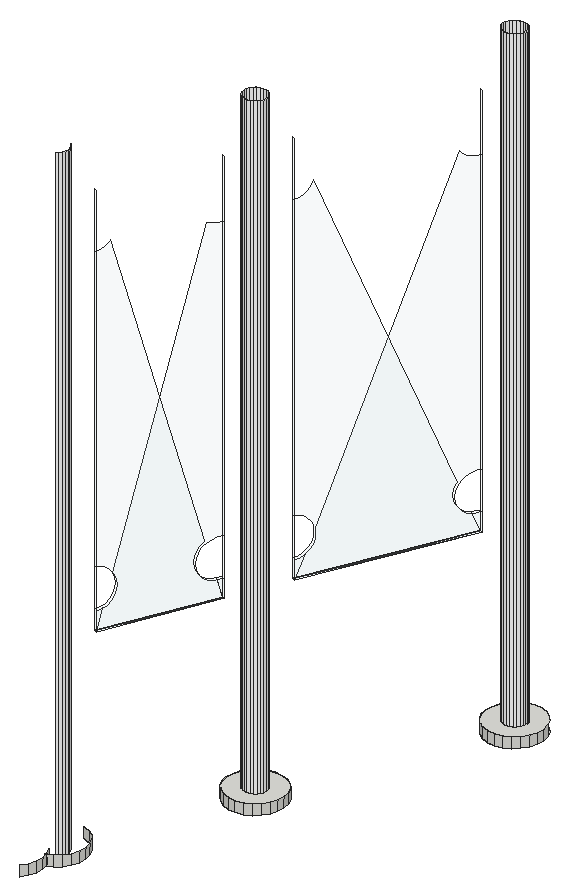
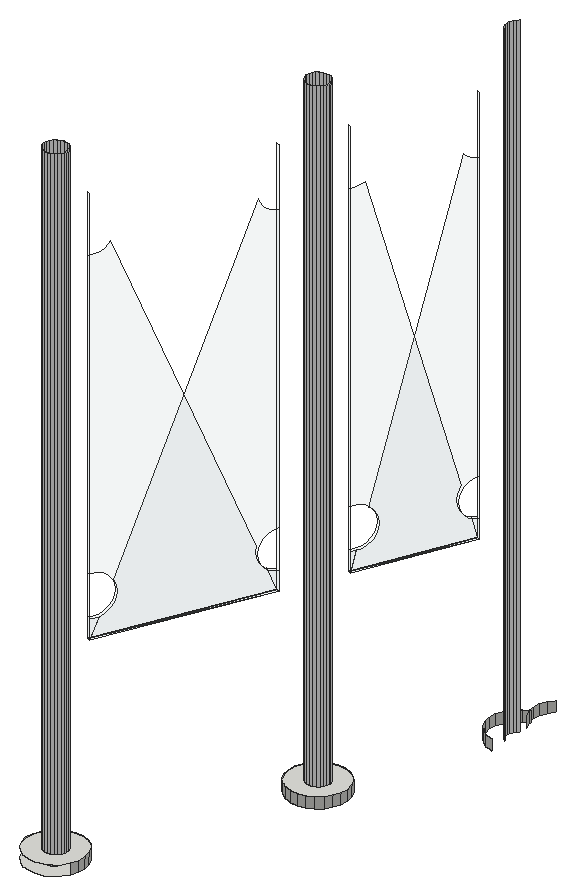
# SketchUp Ruby script. Lengths in inches.
U = 1.inch
M = Sketchup.active_model
def pt(a) = Geom::Point3d.new(a.map { |v| v * U })
def face(e, loops, mat)
  f = e.add_face(loops[0].map { |a| pt(a) })
  loops[1..].each { |l| e.add_face(l.map { |a| pt(a) }).erase! }
  f.material = f.back_material = mat if mat
  f
end
# faces: each face lists its corners as indices into pts; further lists are holes
def faces(e, pts, list, mat = nil) = list.each { |f| face(e, (f[0].is_a?(Array) ? f : [f]).map { |l| l.map { |i| pts[i] } }, mat) }
# xy, xz, yz: faces in a plane at the given z, y or x. An outline is a flat list of corners, or four numbers for a rectangle; further outlines are holes
def ring(l) = l.size == 4 ? [[l[0], l[1]], [l[2], l[1]], [l[2], l[3]], [l[0], l[3]]] : l.each_slice(2).to_a
def flat(e, list, mat, &to3) = list.each { |f| face(e, (f[0].is_a?(Array) ? f : [f]).map { |l| ring(l).map { |u, v| to3.(u, v) } }, mat) }
def xy(e, z, list, mat = nil) = flat(e, list, mat) { |x, y| [x, y, z] }
def xz(e, y, list, mat = nil) = flat(e, list, mat) { |x, z| [x, y, z] }
def yz(e, x, list, mat = nil) = flat(e, list, mat) { |y, z| [x, y, z] }
def lines(e, pts, list) = list.each { |a, b| e.add_line(pt(pts[a]), pt(pts[b])) }
# prism: a flat outline (further loops are holes) pulled along v
def prism(e, loops, v, mat = nil)
  f = face(e, loops, mat); d = Geom::Vector3d.new(v.map { |x| x * U })
  f.pushpull(f.normal.samedirection?(d) ? d.length : -d.length)
end
def box(e, o, s, mat = nil) = prism(e, [[o, [o[0] + s[0], o[1], o[2]], [o[0] + s[0], o[1] + s[1], o[2]], [o[0], o[1] + s[1], o[2]]]], [0, 0, s[2]], mat)
def at(x, y, z, deg = 0) = Geom::Transformation.translation(pt([x, y, z])) * Geom::Transformation.rotation(ORIGIN, Z_AXIS, deg.degrees)
def axes(o, x, y, z) = Geom::Transformation.new([*x, 0, *y, 0, *z, 0, *pt(o).to_a, 1])
def part(name) = M.definitions.add(name)
# library, detail: a bought-in or finely detailed component or shape, given as its bounding box
def library(name, o, s) = part(name).tap { |d| box(d.entities, o, s) }
def detail(e, o, s) = box(e.add_group.entities, o, s)
def put(e, d, t, mat = nil) = e.add_instance(d, t).tap { |i| i.material = mat if mat }
def group(e, t, mat = nil) = e.add_group.tap { |g| g.transformation = t; g.material = mat if mat }.entities
root = M.entities
M.materials.add("Glass_Safety_01").color = [204, 235, 244]
M.materials["Glass_Safety_01"].alpha = 0.1
M.materials.add("[Color_000]").color = [255, 255, 255]
xy(root,321.27,[[[848.125,545.34,848.53,545.42,848.9,545.6,849.2,545.875,849.43,546.22,849.56,546.61,849.58,547.02,849.5,547.42,849.32,547.79,849.05,548.1,848.7,548.32,848.64,548.34,848.3125,548.45,847.9,548.48,847.5,548.4,847.13,548.21,846.82,547.9375,846.6,547.6,846.47,547.21,846.44,546.79,846.53,546.39,846.71,546.02,846.98,545.72,847.33,545.49,847.72,545.36],[848.06,546.28,847.89,546.29,847.76,546.33,847.74,546.34,847.6,546.43,847.49,546.55,847.42,546.7,847.39,546.86,847.4,547.03,847.45,547.18,847.54,547.32,847.66,547.43,847.81,547.5,847.97,547.54,848.13,547.53,848.26,547.48,848.29,547.47,848.43,547.38,848.54,547.26,848.61,547.11,848.64,546.95,848.63,546.79,848.58,546.63,848.49,546.49,848.37,546.39,848.22,546.3125]],[847.39,545.47,847.76,546.33,847.74,546.34,847.6,546.43,847.49,546.55,847.42,546.7,847.39,546.86,847.4,547.03,847.45,547.18,847.54,547.32,847.66,547.43,847.81,547.5,847.97,547.54,848.13,547.53,848.26,547.48,848.64,548.34,848.3125,548.45,847.9,548.48,847.5,548.4,847.13,548.21,846.82,547.9375,846.6,547.6,846.47,547.21,846.44,546.79,846.53,546.39,846.71,546.02,846.98,545.72,847.33,545.49],[847.76,546.33,848.26,547.48,848.13,547.53,847.97,547.54,847.81,547.5,847.66,547.43,847.54,547.32,847.45,547.18,847.4,547.03,847.39,546.86,847.42,546.7,847.49,546.55,847.6,546.43,847.74,546.34],[[853.35,557.32,853.75,557.4,854.12,557.59,854.42,557.86,854.65,558.2,854.78,558.59,854.8,559,854.72,559.41,854.54,559.77,854.26,560.08,853.92,560.31,853.86,560.33,853.53,560.4375,853.12,560.46,852.72,560.38,852.35,560.19,852.04,559.92,851.82,559.58,851.6875,559.1875,851.66,558.78,851.75,558.375,851.93,558.01,852.2,557.7,852.55,557.47,852.94,557.34],[853.28,558.26,853.11,558.27,852.98,558.32,852.96,558.32,852.82,558.41,852.71,558.54,852.64,558.68,852.6,558.85,852.61,559.01,852.67,559.17,852.76,559.3,852.88,559.41,853.03,559.49,853.1875,559.52,853.35,559.51,853.48,559.47,853.51,559.46,853.65,559.37,853.75,559.24,853.83,559.1,853.86,558.9375,853.85,558.77,853.8,558.62,853.71,558.48,853.59,558.37,853.4375,558.3]],[852.61,557.45,852.98,558.32,852.96,558.32,852.82,558.41,852.71,558.54,852.64,558.68,852.6,558.85,852.61,559.01,852.67,559.17,852.76,559.3,852.88,559.41,853.03,559.49,853.1875,559.52,853.35,559.51,853.48,559.47,853.86,560.33,853.53,560.4375,853.12,560.46,852.72,560.38,852.35,560.19,852.04,559.92,851.82,559.58,851.6875,559.1875,851.66,558.78,851.75,558.375,851.93,558.01,852.2,557.7,852.55,557.47],
  [852.96,558.32,852.98,558.32,853.48,559.47,853.35,559.51,853.1875,559.52,853.03,559.49,852.88,559.41,852.76,559.3,852.67,559.17,852.61,559.01,852.6,558.85,852.64,558.68,852.71,558.54,852.82,558.41]])
xy(root,321.27,[[848.06,546.28,848.22,546.3125,848.37,546.39,848.49,546.49,848.58,546.63,848.63,546.79,848.64,546.95,848.61,547.11,848.54,547.26,848.43,547.38,848.29,547.47,848.26,547.48,847.76,546.33,847.89,546.29],[853.28,558.26,853.4375,558.3,853.59,558.37,853.71,558.48,853.8,558.62,853.85,558.77,853.86,558.9375,853.83,559.1,853.75,559.24,853.65,559.37,853.51,559.46,853.48,559.47,852.98,558.32,853.11,558.27]],"[Color_000]")
xy(root,321.86,[[848.125,545.34,848.53,545.42,848.9,545.6,849.2,545.875,849.43,546.22,849.56,546.61,849.58,547.02,849.5,547.42,849.32,547.79,849.05,548.1,848.7,548.32,848.3125,548.45,847.9,548.48,847.5,548.4,847.13,548.21,846.82,547.9375,846.6,547.6,846.47,547.21,846.44,546.79,846.53,546.39,846.71,546.02,846.98,545.72,847.33,545.49,847.72,545.36],[853.35,557.32,853.75,557.4,854.12,557.59,854.42,557.86,854.65,558.2,854.78,558.59,854.8,559,854.72,559.41,854.54,559.77,854.26,560.08,853.92,560.31,853.53,560.4375,853.12,560.46,852.72,560.38,852.35,560.19,852.04,559.92,851.82,559.58,851.6875,559.1875,851.66,558.78,851.75,558.375,851.93,558.01,852.2,557.7,852.55,557.47,852.94,557.34]])
xy(root,331.9,[[844.9,539.5,844.72,539.58,847.47,545.42],[844.72,539.58,847.29,545.5,847.47,545.42],[848.89,548.67,848.71,548.75,852.66,557.32],[848.71,548.75,852.48,557.4,852.66,557.32]],"Glass_Safety_01")
p = [[844.27,534.8,321.27],[844.5,535.14,321.27],[844.5,535.14,321.86],[844.27,534.8,321.86],[844.63,535.53,321.27],[844.63,535.53,321.86],
  [844.66,535.94,321.27],[844.66,535.94,321.86],[844.59,536.27,321.27],[844.57,536.34,321.27],[844.57,536.34,321.86],[844.59,536.27,321.86],
  [844.53,536.25,321.27],[844.9,536.43,321.27],[844.9,536.43,321.86],[844.53,536.25,321.86],[844.39,536.71,321.27],[844.39,536.71,321.86],
  [845.21,536.7,321.27],[845.21,536.7,321.86],[845.4375,537.05,321.27],[845.4375,537.05,321.86],[845.57,537.4375,321.27],[845.57,537.4375,321.86],
  [844.37,537.21,321.27],[844.5,537.32,321.27],[844.5,537.32,357.27],[844.37,537.21,357.27],[844.59,537.46,321.27],[844.59,537.46,357.27],
  [845.59,537.85,321.27],[845.59,537.85,321.86],[844.64,537.62,321.27],[844.64,537.62,357.27],[844.65,537.78,321.27],[844.65,537.78,357.27],
  [844.61,537.94,321.27],[844.61,537.94,357.27],[845.51,538.25,321.27],[845.51,538.25,321.86],[844.54,538.09,321.27],[844.54,538.09,357.27],
  [844.43,538.21,321.27],[844.43,538.21,357.27],[845.32,538.62,321.27],[845.32,538.62,321.86],[845.05,538.93,321.27],[845.05,538.93,321.86],
  [844.71,539.15,321.27],[844.71,539.15,321.86],[844.65,539.17,321.27],[844.32,539.28,321.27],[844.32,539.28,321.86],[847.72,545.36,321.27],
  [848.125,545.34,321.27],[848.125,545.34,321.86],[847.72,545.36,321.86],[848.53,545.42,321.27],[848.53,545.42,321.86],[847.33,545.49,321.27],
  [847.39,545.47,321.27],[847.33,545.49,321.86],[848.9,545.6,321.27],[848.9,545.6,321.86],[846.98,545.72,321.27],[846.98,545.72,321.86],
  [849.2,545.875,321.27],[849.2,545.875,321.86],[846.71,546.02,321.27],[846.71,546.02,321.86],[849.43,546.22,321.27],[849.43,546.22,321.86],
  [846.53,546.39,321.27],[846.53,546.39,321.86],[849.56,546.61,321.27],[849.56,546.61,321.86],[847.6,546.43,321.27],[847.74,546.34,321.27],
  [847.74,546.34,357.27],[847.6,546.43,357.27],[847.76,546.33,321.27],[847.89,546.29,321.27],[847.89,546.29,357.27],[848.06,546.28,321.27],
  [848.06,546.28,357.27],[848.22,546.3125,321.27],[848.22,546.3125,357.27],[848.37,546.39,321.27],[848.37,546.39,357.27],[846.44,546.79,321.27],
  [846.44,546.79,321.86],[847.49,546.55,321.27],[847.49,546.55,357.27],[848.49,546.49,321.27],[848.49,546.49,357.27],[848.58,546.63,321.27],
  [848.58,546.63,357.27],[847.42,546.7,321.27],[847.42,546.7,357.27],[848.63,546.79,321.27],[848.63,546.79,357.27],[849.58,547.02,321.27],
  [849.58,547.02,321.86],[847.39,546.86,321.27],[847.39,546.86,357.27],[846.47,547.21,321.27],[846.47,547.21,321.86],[848.64,546.95,321.27],
  [848.64,546.95,357.27],[847.4,547.03,321.27],[847.4,547.03,357.27],[847.45,547.18,321.27],[847.45,547.18,357.27],[848.61,547.11,321.27],
  [848.61,547.11,357.27],[849.5,547.42,321.27],[849.5,547.42,321.86],[848.54,547.26,321.27],[848.54,547.26,357.27],[846.6,547.6,321.27],
  [846.6,547.6,321.86],[847.54,547.32,321.27],[847.54,547.32,357.27],[847.66,547.43,321.27],[847.66,547.43,357.27],[848.43,547.38,321.27],
  [848.43,547.38,357.27],[847.81,547.5,321.27],[847.81,547.5,357.27],[848.29,547.47,321.27],[848.29,547.47,357.27],[849.32,547.79,321.27],
  [849.32,547.79,321.86],[847.97,547.54,321.27],[847.97,547.54,357.27],[848.13,547.53,321.27],[848.13,547.53,357.27],[848.26,547.48,321.27],
  [846.82,547.9375,321.27],[846.82,547.9375,321.86],[849.05,548.1,321.27],[849.05,548.1,321.86],[847.13,548.21,321.27],[847.13,548.21,321.86],
  [848.7,548.32,321.27],[848.7,548.32,321.86],[847.5,548.4,321.27],[847.5,548.4,321.86],[848.64,548.34,321.27],[848.3125,548.45,321.27],
  [848.3125,548.45,321.86],[847.9,548.48,321.27],[847.9,548.48,321.86],[852.55,557.47,321.27],[852.61,557.45,321.27],[852.94,557.34,321.27],
  [852.94,557.34,321.86],[852.55,557.47,321.86],[853.35,557.32,321.27],[853.35,557.32,321.86],[853.75,557.4,321.27],[853.75,557.4,321.86],
  [854.12,557.59,321.27],[854.12,557.59,321.86],[852.2,557.7,321.27],[852.2,557.7,321.86],[854.42,557.86,321.27],[854.42,557.86,321.86],
  [851.93,558.01,321.27],[851.93,558.01,321.86],[854.65,558.2,321.27],[854.65,558.2,321.86],[851.75,558.375,321.27],[851.75,558.375,321.86],
  [854.78,558.59,321.27],[854.78,558.59,321.86],[852.82,558.41,321.27],[852.96,558.32,321.27],[852.96,558.32,357.27],[852.82,558.41,357.27],
  [852.98,558.32,321.27],[853.11,558.27,321.27],[853.11,558.27,357.27],[853.28,558.26,321.27],[853.28,558.26,357.27],[853.4375,558.3,321.27],
  [853.4375,558.3,357.27],[853.59,558.37,321.27],[853.59,558.37,357.27],[851.66,558.78,321.27],[851.66,558.78,321.86],[852.71,558.54,321.27],
  [852.71,558.54,357.27],[853.71,558.48,321.27],[853.71,558.48,357.27],[852.64,558.68,321.27],[852.64,558.68,357.27],[853.8,558.62,321.27],
  [853.8,558.62,357.27],[853.85,558.77,321.27],[853.85,558.77,357.27],[854.8,559,321.27],[854.8,559,321.86],[852.6,558.85,321.27],
  [852.6,558.85,357.27],[851.6875,559.1875,321.27],[851.6875,559.1875,321.86],[852.61,559.01,321.27],[852.61,559.01,357.27],[853.86,558.9375,321.27],
  [853.86,558.9375,357.27],[853.83,559.1,321.27],[853.83,559.1,357.27],[852.67,559.17,321.27],[852.67,559.17,357.27],[854.72,559.41,321.27],
  [854.72,559.41,321.86],[853.75,559.24,321.27],[853.75,559.24,357.27],[851.82,559.58,321.27],[851.82,559.58,321.86],[852.76,559.3,321.27],
  [852.76,559.3,357.27],[853.65,559.37,321.27],[853.65,559.37,357.27],[852.88,559.41,321.27],[852.88,559.41,357.27],[853.03,559.49,321.27],
  [853.03,559.49,357.27],[853.51,559.46,321.27],[853.51,559.46,357.27],[853.1875,559.52,321.27],[853.1875,559.52,357.27],[853.35,559.51,321.27],
  [853.35,559.51,357.27],[853.48,559.47,321.27],[844.72,539.58,331.9],[844.9,539.5,331.9],[844.9,539.5,333],[844.9,539.5,335.125],
  [844.9,539.5,351.28],[844.9,539.5,353.41],[844.9,539.5,354.51],[844.72,539.58,354.51],[844.72,539.58,353.41],[844.72,539.58,351.28],
  [844.72,539.58,335.125],[844.72,539.58,333],[845.03,539.8,333.06],[845.01,539.75,333.04],[847.47,545.42,335.125],[847.47,545.42,351.28],
  [847.32,545.0625,351.28],[847.21,544.8125,351.32],[847.12,544.61,351.41],[845.22,540.24,334.74],[845.26,540.34,334.59],[845.31,540.44,334.34],
  [845.32,540.48,334.0625],[845.31,540.44,333.79],[845.26,540.34,333.53],[845.2,540.19,333.3125],[845.11,539.99,333.14],[847.47,545.42,331.9],
  [847.47,545.42,333],[847.32,545.0625,333],[847.21,544.8125,333.04],[847.11,544.58,333.14],[847.02,544.375,333.3125],[846.95,544.22,333.53],
  [846.91,544.12,333.79],[846.89,544.09,334.0625],[846.91,544.12,334.34],[846.95,544.22,334.59],[847.02,544.375,334.8125],[847.11,544.58,334.98],
  [847.21,544.8125,335.09],[847.32,545.0625,335.125],[844.83,539.83,351.32],[844.93,540.07,351.43],[845.02,540.27,351.59],[845.04,540.32,351.67],
  [846.9375,544.6875,335],[846.93,544.65,334.98],[846.84,544.45,334.8125],[846.77,544.3,334.59],[846.73,544.2,334.34],[846.71,544.17,334.0625],
  [846.73,544.2,333.79],[846.77,544.3,333.53],[846.84,544.45,333.3125],[846.93,544.65,333.14],[847.03,544.89,333.04],[847.14,545.14,333],
  [847.17,545.21,333],[847.29,545.5,331.9],[844.83,539.83,333.04],[844.93,540.07,333.14],[845.02,540.27,333.3125],[845.08,540.42,333.53],
  [845.125,540.52,333.79],[845.14,540.55,334.0625],[845.125,540.52,334.34],[845.08,540.42,334.59],[845.02,540.27,334.8125],[844.93,540.07,334.98],
  [844.83,539.83,335.09],[847.29,545.5,333],[847.29,545.5,335.125],[847.29,545.5,351.28],[847.29,545.5,353.41],[847.29,545.5,354.51],
  [847.47,545.42,354.51],[847.47,545.42,353.41],[848.71,548.75,331.9],[848.89,548.67,331.9],[848.89,548.67,333],[848.89,548.67,335.125],
  [848.89,548.67,351.28],[848.89,548.67,353.41],[848.89,548.67,354.51],[848.71,548.75,354.51],[848.71,548.75,353.41],[848.71,548.75,351.28],
  [848.71,548.75,335.125],[848.71,548.75,333],[849.1,549.15,333.14],[849,548.92,333.04],[852.66,557.32,335.125],[852.66,557.32,351.28],
  [852.54,557.05,351.28],[852.43,556.79,351.32],[852.33,556.56,351.43],[852.24,556.36,351.59],[852.19,556.26,351.74],[849.3,549.61,334.35],
  [849.3,549.61,334.34],[849.31,549.65,334.0625],[849.3,549.61,333.79],[849.26,549.52,333.53],[849.19,549.36,333.3125],[849.1,549.16,333.14],
  [852.66,557.32,331.9],[852.66,557.32,333],[852.54,557.05,333],[852.43,556.79,333.04],[852.33,556.56,333.14],[852.24,556.36,333.3125],
  [852.17,556.2,333.53],[852.13,556.11,333.79],[852.11,556.07,334.0625],[852.13,556.11,334.34],[852.17,556.2,334.59],[852.24,556.36,334.8125],
  [852.33,556.56,334.98],[852.43,556.79,335.09],[852.54,557.05,335.125],[849.12,549.6875,352.06],[852.01,556.34,334.67],[851.99,556.28,334.59],
  [851.95,556.18,334.34],[851.93,556.15,334.0625],[851.95,556.18,333.79],[851.99,556.28,333.53],[852.06,556.4375,333.3125],[852.14,556.64,333.14],
  [852.25,556.87,333.04],[852.29,556.97,333.02],[852.48,557.4,331.9],[848.82,549,333.04],[848.92,549.24,333.14],[849.01,549.44,333.3125],
  [849.08,549.6,333.53],[849.12,549.69,333.79],[849.13,549.73,334.0625],[849.12,549.69,334.34],[849.08,549.6,334.59],[849.01,549.44,334.8125],
  [848.92,549.24,334.98],[848.82,549,335.09],[848.82,549,351.32],[848.92,549.24,351.43],[849.01,549.44,351.59],[849.08,549.6,351.81],
  [852.36,557.125,333],[852.48,557.4,333],[852.48,557.4,335.125],[852.48,557.4,351.28],[852.48,557.4,353.41],[852.48,557.4,354.51],
  [852.66,557.32,354.51],[852.66,557.32,353.41]]
faces(root,p,[[0,1,2,3],[1,4,5,2],[4,6,7,5],[6,8,9,10,11,7],[12,8,13,14,11,15],[9,16,17,10],[13,18,19,14],[18,20,21,19],
  [20,22,23,21],[22,30,31,23],[30,38,39,31],[38,44,45,39],[44,46,47,45],[46,48,49,47],[48,50,51,52,49],[53,54,55,56],
  [54,57,58,55],[59,60,53,56,61],[57,62,63,58],[64,59,61,65],[62,66,67,63],[68,64,65,69],[66,70,71,67],[72,68,69,73],
  [70,74,75,71],[89,72,73,90],[74,101,102,75],[105,89,90,106],[101,115,116,102],[119,105,106,120],[115,131,132,116],[138,119,120,139],
  [131,140,141,132],[142,138,139,143],[140,144,145,141],[146,142,143,147],[144,148,149,150,145],[151,146,147,152],[149,151,152,150],[153,154,155,156,157],
  [155,158,159,156],[158,160,161,159],[160,162,163,161],[164,153,157,165],[162,166,167,163],[168,164,165,169],[166,170,171,167],[172,168,169,173],
  [170,174,175,171],[189,172,173,190],[174,201,202,175],[205,189,190,206],[201,215,216,202],[219,205,206,220]])
faces(root,p,[[24,25,26,27],[25,28,29,26],[28,32,33,29],[32,34,35,33],[34,36,37,35],[36,40,41,37],[40,42,43,41],[76,77,78,79],
  [77,80,81,82,78],[81,83,84,82],[83,85,86,84],[85,87,88,86],[91,76,79,92],[87,93,94,88],[93,95,96,94],[97,91,92,98],
  [95,99,100,96],[103,97,98,104],[99,107,108,100],[109,103,104,110],[111,109,110,112],[107,113,114,108],[113,117,118,114],[121,111,112,122],
  [123,121,122,124],[117,125,126,118],[127,123,124,128],[125,129,130,126],[133,127,128,134],[135,133,134,136],[129,137,135,136,130],[176,177,178,179],
  [177,180,181,182,178],[181,183,184,182],[183,185,186,184],[185,187,188,186],[191,176,179,192],[187,193,194,188],[195,191,192,196],[193,197,198,194],
  [197,199,200,198],[203,195,196,204],[207,203,204,208],[199,209,210,200],[209,211,212,210],[213,207,208,214],[211,217,218,212],[221,213,214,222],
  [217,223,224,218],[225,221,222,226],[227,225,226,228],[223,229,230,224],[231,227,228,232],[233,231,232,234],[229,235,233,234,230]],"[Color_000]")
faces(root,p,[[236,237,238,239,240,241,242,243,244,245,246,247],[237,248,249,238],[250,251,252,253,254,255,256,257,258,259,260,261,262,248,237,263,264,265,266,267,268,269,270,271,272,273,274,275,276,277],[246,245,278,279,280,281,282,283,284,285,286,287,288,289,290,291,292,293,294,295,236,247,296,297,298,299,300,301,302,303,304,305,306],[295,294,307],[263,295,307,308,309,310,311,312,313,251,250,264],[314,315,316,317,318,319,320,321,322,323,324,325],[315,326,327,316],
  [328,329,330,331,332,333,334,335,336,337,338,339,340,341,326,315,342,343,344,345,346,347,348,349,350,351,352,353,354,355,356],[357,358,359,360,361,362,363,364,365,366,367,368,314,325,369,370,371,372,373,374,375,376,377,378,379,324,323,380,381,382,383],[368,367,384,385],[342,368,385,386,387,388,389,390,391,329,328,343]],"Glass_Safety_01")
